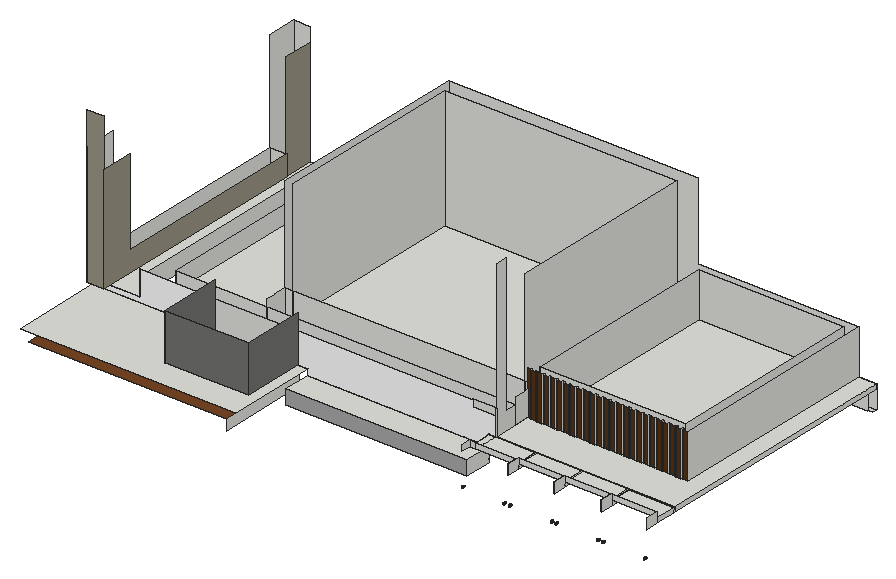
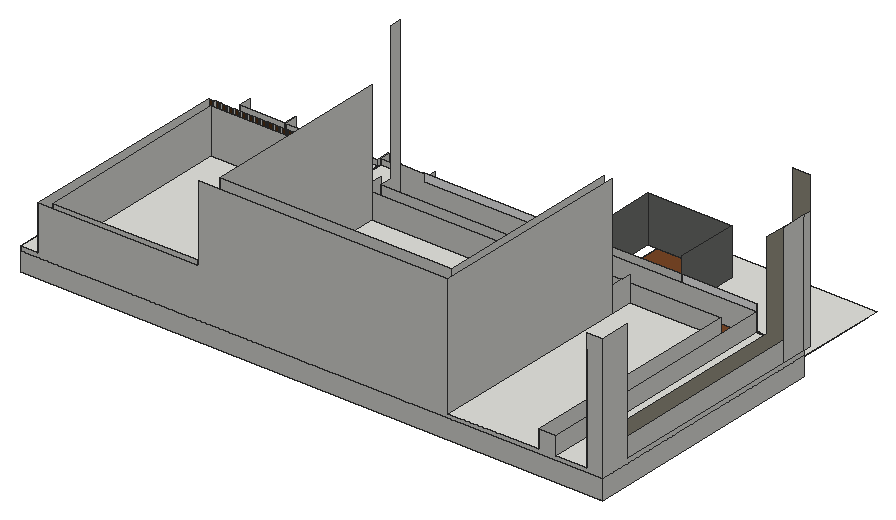
# SketchUp Ruby script. Lengths in inches.
U = 1.inch
M = Sketchup.active_model
def pt(a) = Geom::Point3d.new(a.map { |v| v * U })
def face(e, loops, mat)
  f = e.add_face(loops[0].map { |a| pt(a) })
  loops[1..].each { |l| e.add_face(l.map { |a| pt(a) }).erase! }
  f.material = f.back_material = mat if mat
  f
end
# faces: each face lists its corners as indices into pts; further lists are holes
def faces(e, pts, list, mat = nil) = list.each { |f| face(e, (f[0].is_a?(Array) ? f : [f]).map { |l| l.map { |i| pts[i] } }, mat) }
# xy, xz, yz: faces in a plane at the given z, y or x. An outline is a flat list of corners, or four numbers for a rectangle; further outlines are holes
def ring(l) = l.size == 4 ? [[l[0], l[1]], [l[2], l[1]], [l[2], l[3]], [l[0], l[3]]] : l.each_slice(2).to_a
def flat(e, list, mat, &to3) = list.each { |f| face(e, (f[0].is_a?(Array) ? f : [f]).map { |l| ring(l).map { |u, v| to3.(u, v) } }, mat) }
def xy(e, z, list, mat = nil) = flat(e, list, mat) { |x, y| [x, y, z] }
def xz(e, y, list, mat = nil) = flat(e, list, mat) { |x, z| [x, y, z] }
def yz(e, x, list, mat = nil) = flat(e, list, mat) { |y, z| [x, y, z] }
def lines(e, pts, list) = list.each { |a, b| e.add_line(pt(pts[a]), pt(pts[b])) }
# prism: a flat outline (further loops are holes) pulled along v
def prism(e, loops, v, mat = nil)
  f = face(e, loops, mat); d = Geom::Vector3d.new(v.map { |x| x * U })
  f.pushpull(f.normal.samedirection?(d) ? d.length : -d.length)
end
def box(e, o, s, mat = nil) = prism(e, [[o, [o[0] + s[0], o[1], o[2]], [o[0] + s[0], o[1] + s[1], o[2]], [o[0], o[1] + s[1], o[2]]]], [0, 0, s[2]], mat)
def at(x, y, z, deg = 0) = Geom::Transformation.translation(pt([x, y, z])) * Geom::Transformation.rotation(ORIGIN, Z_AXIS, deg.degrees)
def axes(o, x, y, z) = Geom::Transformation.new([*x, 0, *y, 0, *z, 0, *pt(o).to_a, 1])
def part(name) = M.definitions.add(name)
# library, detail: a bought-in or finely detailed component or shape, given as its bounding box
def library(name, o, s) = part(name).tap { |d| box(d.entities, o, s) }
def detail(e, o, s) = box(e.add_group.entities, o, s)
def put(e, d, t, mat = nil) = e.add_instance(d, t).tap { |i| i.material = mat if mat }
def group(e, t, mat = nil) = e.add_group.tap { |g| g.transformation = t; g.material = mat if mat }.entities
root = M.entities
M.materials.add("[0030_OldLace]").color = [86, 53, 24]
M.materials.add("[0128_White]").color = [255, 255, 255]
M.materials.add("[Color M03]").color = [170, 170, 170]
M.materials.add("[Concrete Tile]").color = [155, 150, 134]
M.materials.add("[Metal Seamed]").color = [116, 117, 113]
M.materials.add("[Wood Veneer 01]").color = [120, 70, 37]
xy(root,95.79,[[1564.1,846.1,1664.38,851.0625]])
xy(root,99.26,[[1501.42,810.97,1728.67,845.35]],"[Wood Veneer 01]")
xy(root,101.375,[[1425.1,845.35,1490.48,846.1],[1232.12,846.1,1232.12,1160.85,1960.87,1160.85,1960.87,1155.13,1237.84,1155.13,1237.84,851.0625,1425.1,851.0625,1425.1,846.1],[1425.1,846.1,1490.48,851.0625]])
xy(root,101.78,[[1254.78,845.35,1379.65,851.0625]])
xy(root,114.25,[[1243.06,732.28,1490.48,845.35]],"[Wood Veneer 01]")
xy(root,117.26,[[1501.42,810.97,1728.67,845.35]])
xy(root,125.1875,[[1232.12,732.28,1501.42,732.28,1501.42,845.35,1489.48,845.35,1489.48,767.72,1385.29,767.72,1385.29,845.35,1232.12,845.35],[1232.12,845.35,1501.42,846.1]])
xy(root,131.1875,[[1728.67,814.22,1729.13,844.47],[1729.13,814.22,1737.07,844.47],[1737.07,814.22,1786.72,844.47],[1787.65,817.6,1844.77,844.47],[1845.83,817.6,1902.82,844.47],
  [1904.13,817.6,1960.87,844.47],[1232.12,837.03,1252.87,845.35],[1728.67,844.47,1729.13,845.35],[1729.13,844.47,1737.07,845.35],[1737.07,844.47,1960.87,846.1],
  [1232.12,845.35,1252.87,846.1],[1252.87,845.35,1291.04,846.1],[1728.67,845.35,1729.13,846.1],[1729.13,845.35,1737.07,846.1],[1232.12,846.1,1252.87,877.14],
  [1252.87,846.1,1291.04,846.1,1291.04,1160.85,1252.24,1160.85,1252.24,1122.97,1252.87,1122.97],[1737.07,846.1,1960.87,846.1,1960.87,1160.85,1938.44,1160.85,1938.44,893.65,1932.29,893.65,1932.29,895.71,1930.13,895.71,1930.13,893.65,1923.98,893.65,1923.98,895.71,1921.82,895.71,1921.82,894.34,1915.67,894.34,1915.67,895.71,1913.51,895.71,1913.51,894.34,1907.36,894.34,1907.36,895.71,1905.19,895.71,1905.19,894.34,1899.04,894.34,1899.04,895.71,1896.88,895.71,1896.88,894.34,1890.73,894.34,1890.73,895.71,1888.57,895.71,1888.57,894.34,1882.42,894.34,1882.42,895.71,1880.26,895.71,1880.26,894.34,1874.11,894.34,1874.11,895.71,1871.94,895.71,1871.94,894.34,1865.79,894.34,1865.79,895.71,1863.63,895.71,1863.63,894.34,1857.48,894.34,1857.48,895.71,1855.32,895.71,1855.32,894.34,1849.17,894.34,1849.17,895.71,1847.01,895.71,1847.01,894.34,1840.86,894.34,1840.86,895.71,1838.69,895.71,1838.69,894.34,1832.54,894.34,1832.54,895.71,1830.38,895.71,1830.38,894.34,1824.23,894.34,1824.23,895.71,1822.07,895.71,1822.07,894.34,1815.92,894.34,1815.92,895.71,1813.76,895.71,1813.76,894.34,1807.61,894.34,1807.61,895.71,1805.44,895.71,1805.44,894.34,1799.29,894.34,1799.29,895.71,1797.13,895.71,1797.13,894.34,1790.98,894.34,1790.98,895.71,1788.82,895.71,1788.82,894.34,1782.67,894.34,1782.67,895.71,1780.51,895.71,1780.51,894.34,1774.36,894.34,1774.36,895.71,1772.19,895.71,1772.19,894.34,1766.04,894.34,1766.04,895.71,1763.88,895.71,1763.88,894.34,1757.73,894.34,1757.73,895.71,1755.57,895.71,1755.57,894.34,1749.42,894.34,1749.42,895.71,1747.26,895.71,1747.26,894.34,1741.11,894.34,1741.11,895.71,1737.07,895.71],[1232.12,877.14,1252.87,1122.97],[1311.45,877.14,1425.1,1160.85],[1425.1,877.14,1737.07,905.7],
  [1745.54,904.18,1927.22,1152.375],[1434.48,905.7,1724.81,1143.26]])
xz(root,767.72,[[1385.29,125.1875,1489.48,183.3125]],"[Metal Seamed]")
xz(root,799.91,[[1731.49,91.63,1731.78,91.67,1732.05,91.78,1732.29,91.96,1732.46,92.19,1732.58,92.46,1732.61,92.75,1732.58,93.04,1732.46,93.32,1732.29,93.55,1732.05,93.73,1731.78,93.84,1731.49,93.88,1731.2,93.84,1730.93,93.73,1730.69,93.55,1730.52,93.32,1730.4,93.04,1730.36,92.75,1730.4,92.46,1730.52,92.19,1730.69,91.96,1730.93,91.78,1731.2,91.67],[1783.68,91.63,1783.97,91.67,1784.24,91.78,1784.47,91.96,1784.65,92.19,1784.76,92.46,1784.8,92.75,1784.76,93.04,1784.65,93.32,1784.47,93.55,1784.24,93.73,1783.97,93.84,1783.68,93.88,1783.39,93.84,1783.11,93.73,1782.88,93.55,1782.7,93.32,1782.59,93.04,1782.55,92.75,1782.59,92.46,1782.7,92.19,1782.88,91.96,1783.11,91.78,1783.39,91.67],[1790.48,91.63,1790.77,91.67,1791.04,91.78,1791.27,91.96,1791.45,92.19,1791.56,92.46,1791.6,92.75,1791.56,93.04,1791.45,93.32,1791.27,93.55,1791.04,93.73,1790.77,93.84,1790.48,93.88,1790.1875,93.84,1789.92,93.73,1789.68,93.55,1789.5,93.32,1789.39,93.04,1789.35,92.75,1789.39,92.46,1789.5,92.19,1789.68,91.96,1789.92,91.78,1790.1875,91.67],[1842.67,91.63,1842.96,91.67,1843.23,91.78,1843.46,91.96,1843.64,92.19,1843.75,92.46,1843.79,92.75,1843.75,93.04,1843.64,93.32,1843.46,93.55,1843.23,93.73,1842.96,93.84,1842.67,93.88,1842.375,93.84,1842.1,93.73,1841.87,93.55,1841.69,93.32,1841.58,93.04,1841.54,92.75,1841.58,92.46,1841.69,92.19,1841.87,91.96,1842.1,91.78,1842.375,91.67],[1848.65,91.63,1848.94,91.67,1849.22,91.78,1849.45,91.96,1849.63,92.19,1849.74,92.46,1849.78,92.75,1849.74,93.04,1849.63,93.32,1849.45,93.55,1849.22,93.73,1848.94,93.84,1848.65,93.88,1848.36,93.84,1848.09,93.73,1847.86,93.55,1847.68,93.32,1847.57,93.04,1847.53,92.75,1847.57,92.46,1847.68,92.19,1847.86,91.96,1848.09,91.78,1848.36,91.67],
  [1900.84,91.63,1901.13,91.67,1901.4,91.78,1901.64,91.96,1901.82,92.19,1901.93,92.46,1901.97,92.75,1901.93,93.04,1901.82,93.32,1901.64,93.55,1901.4,93.73,1901.13,93.84,1900.84,93.88,1900.55,93.84,1900.28,93.73,1900.05,93.55,1899.87,93.32,1899.75,93.04,1899.72,92.75,1899.75,92.46,1899.87,92.19,1900.05,91.96,1900.28,91.78,1900.55,91.67],[1906.95,91.63,1907.25,91.67,1907.52,91.78,1907.75,91.96,1907.93,92.19,1908.04,92.46,1908.08,92.75,1908.04,93.04,1907.93,93.32,1907.75,93.55,1907.52,93.73,1907.25,93.84,1906.95,93.88,1906.66,93.84,1906.39,93.73,1906.16,93.55,1905.98,93.32,1905.87,93.04,1905.83,92.75,1905.87,92.46,1905.98,92.19,1906.16,91.96,1906.39,91.78,1906.66,91.67],[1959.14,91.63,1959.43,91.67,1959.7,91.78,1959.9375,91.96,1960.12,92.19,1960.23,92.46,1960.27,92.75,1960.23,93.04,1960.12,93.32,1959.9375,93.55,1959.7,93.73,1959.43,93.84,1959.14,93.88,1958.85,93.84,1958.58,93.73,1958.35,93.55,1958.17,93.32,1958.06,93.04,1958.02,92.75,1958.06,92.46,1958.17,92.19,1958.35,91.96,1958.58,91.78,1958.85,91.67]])
xz(root,810.97,[[1501.42,99.26,1728.67,117.26]],"[Color M03]")
xz(root,814.22,[[1728.67,131.1875,1737.07,138.0625],[1737.07,131.1875,1786.72,138.0625]])
xz(root,817.6,[[1787.65,131.1875,1844.77,138.0625],[1845.83,131.1875,1902.82,138.0625],[1904.13,131.1875,1960.87,138.0625]])
xz(root,837.03,[[1232.12,131.1875,1252.87,324.5625]],"[Concrete Tile]")
xz(root,845.35,[[1501.42,99.26,1728.67,117.26],[1385.29,125.1875,1489.48,162.75]])
xz(root,845.35,[[1501.42,117.26,1728.67,117.26,1728.67,131.1875,1737.07,131.1875,1737.07,154.75,1707.86,154.75,1707.86,162.75,1489.48,162.75,1489.48,125.1875,1501.42,125.1875],[1232.12,125.1875,1385.29,125.1875,1385.29,162.75,1291.04,162.75,1291.04,131.1875,1232.12,131.1875]],"[0128_White]")
xz(root,846.1,[[1232.12,125.1875,1232.12,131.1875,1291.04,131.1875,1291.04,153.5625,1707.86,153.5625,1707.86,163,1737.07,163,1737.07,131.1875,1728.67,131.1875,1728.67,125.1875]])
xz(root,851.0625,[[1254.78,101.375,1379.65,101.78]])
xz(root,877.14,[[1311.45,131.1875,1425.1,153.5625],[1425.1,131.1875,1737.07,153.5625]])
xz(root,893.65,[[1923.98,131.1875,1930.13,186.75],[1932.29,131.1875,1938.44,186.75]],"[0030_OldLace]")
xz(root,894.34,[[1741.11,131.1875,1747.26,186.75],[1749.42,131.1875,1755.57,186.75],[1757.73,131.1875,1763.88,186.75],[1766.04,131.1875,1772.19,186.75],[1774.36,131.1875,1780.51,186.75],
  [1782.67,131.1875,1788.82,186.75],[1790.98,131.1875,1797.13,186.75],[1799.29,131.1875,1805.44,186.75],[1807.61,131.1875,1813.76,186.75],[1815.92,131.1875,1822.07,186.75],
  [1824.23,131.1875,1830.38,186.75],[1832.54,131.1875,1838.69,186.75],[1840.86,131.1875,1847.01,186.75],[1849.17,131.1875,1855.32,186.75],[1857.48,131.1875,1863.63,186.75],
  [1865.79,131.1875,1871.94,186.75],[1874.11,131.1875,1880.26,186.75],[1882.42,131.1875,1888.57,186.75],[1890.73,131.1875,1896.88,186.75],[1899.04,131.1875,1905.19,186.75],
  [1907.36,131.1875,1913.51,186.75],[1915.67,131.1875,1921.82,186.75]],"[0030_OldLace]")
xz(root,895.71,[[1737.07,131.1875,1741.11,186.75],[1747.26,131.1875,1749.42,186.75],[1755.57,131.1875,1757.73,186.75],[1763.88,131.1875,1766.04,186.75],[1772.19,131.1875,1774.36,186.75],
  [1780.51,131.1875,1782.67,186.75],[1788.82,131.1875,1790.98,186.75],[1797.13,131.1875,1799.29,186.75],[1805.44,131.1875,1807.61,186.75],[1813.76,131.1875,1815.92,186.75],
  [1822.07,131.1875,1824.23,186.75],[1830.38,131.1875,1832.54,186.75],[1838.69,131.1875,1840.86,186.75],[1847.01,131.1875,1849.17,186.75],[1855.32,131.1875,1857.48,186.75],
  [1863.63,131.1875,1865.79,186.75],[1871.94,131.1875,1874.11,186.75],[1880.26,131.1875,1882.42,186.75],[1888.57,131.1875,1890.73,186.75],[1896.88,131.1875,1899.04,186.75],
  [1905.19,131.1875,1907.36,186.75],[1913.51,131.1875,1915.67,186.75],[1921.82,131.1875,1923.98,186.75],[1930.13,131.1875,1932.29,186.75]],"[0030_OldLace]")
xz(root,904.18,[[1745.54,131.1875,1927.22,186.75]])
xz(root,905.7,[[1425.1,131.1875,1434.48,162.75],[1434.48,131.1875,1724.81,162.75],[1724.81,131.1875,1737.07,162.75]])
xz(root,1122.97,[[1232.12,131.1875,1252.24,156.5],[1252.24,131.1875,1252.87,156.5]])
xz(root,1143.26,[[1434.48,131.1875,1724.81,282.75]])
xz(root,1152.375,[[1745.54,131.1875,1927.22,186.75]])
xz(root,1155.13,[[1237.84,101.375,1955.15,125.1875]])
xz(root,1160.85,[[1232.12,101.375,1960.87,125.1875],[1232.12,125.1875,1232.12,282.75,1252.24,282.75,1252.24,131.1875,1291.04,131.1875,1291.04,153.5625,1311.45,153.5625,1311.45,131.1875,1425.1,131.1875,1425.1,282.75,1737.07,282.75,1737.07,186.75,1938.44,186.75,1938.44,131.1875,1960.87,131.1875,1960.87,125.1875]])
yz(root,1232.12,[[846.1,101.375,1160.85,125.1875],[845.35,125.1875,846.1,131.1875],[846.1,125.1875,846.1,131.1875,1122.97,131.1875,1122.97,282.75,1160.85,282.75,1160.85,125.1875],[837.03,131.1875,845.35,282.75],[845.35,131.1875,877.14,282.75],
  [877.14,131.1875,1122.97,156.5]])
yz(root,1237.84,[[851.0625,101.375,1155.13,125.1875]])
yz(root,1252.24,[[1122.97,131.1875,1160.85,264.75]],"[Concrete Tile]")
yz(root,1252.87,[[837.03,131.1875,1122.97,131.1875,1122.97,156.5,877.14,156.5,877.14,264.75,837.03,264.75]],"[Concrete Tile]")
yz(root,1291.04,[[845.35,131.1875,846.1,162.75],[846.1,131.1875,1160.85,153.5625]])
yz(root,1311.45,[[877.14,131.1875,1160.85,153.5625]])
yz(root,1385.29,[[767.72,125.1875,845.35,183.3125]],"[Metal Seamed]")
yz(root,1425.1,[[877.14,131.1875,877.14,162.125,888.95,162.125,888.95,162.75,905.7,162.75,905.7,131.1875],[905.7,131.1875,1160.85,282.75]])
yz(root,1434.48,[[905.7,131.1875,1143.26,282.75]])
yz(root,1489.48,[[767.72,125.1875,845.35,183.3125]],"[Metal Seamed]")
yz(root,1490.48,[[732.28,101.375,845.35,114.25]])
yz(root,1724.81,[[905.7,131.1875,1143.26,282.75]])
yz(root,1728.67,[[810.97,99.26,844.47,117.26],[844.47,99.26,845.35,117.26],[844.47,117.26,845.35,125.1875],[844.47,125.1875,845.35,131.1875],[845.35,125.1875,846.1,131.1875],
  [801.78,131.1875,814.22,138.0625]])
yz(root,1737.07,[[845.35,131.1875,846.1,163],[846.1,131.1875,877.14,131.1875,877.14,153.5625,861.24,153.5625,861.24,324.5625,846.1,324.5625],[877.14,131.1875,895.71,131.1875,895.71,162.75,890.39,162.75,890.39,162.125,877.14,162.125],[895.71,131.1875,905.7,162.75]])
yz(root,1741.11,[[894.34,131.1875,895.71,186.75]])
yz(root,1745.54,[[904.18,131.1875,905.7,186.75],[905.7,131.1875,1152.375,186.75]])
yz(root,1747.26,[[894.34,131.1875,895.71,186.75]])
yz(root,1749.42,[[894.34,131.1875,895.71,186.75]])
yz(root,1755.57,[[894.34,131.1875,895.71,186.75]])
yz(root,1757.73,[[894.34,131.1875,895.71,186.75]])
yz(root,1763.88,[[894.34,131.1875,895.71,186.75]])
yz(root,1766.04,[[894.34,131.1875,895.71,186.75]])
yz(root,1772.19,[[894.34,131.1875,895.71,186.75]])
yz(root,1774.36,[[894.34,131.1875,895.71,186.75]])
yz(root,1780.51,[[894.34,131.1875,895.71,186.75]])
yz(root,1782.67,[[894.34,131.1875,895.71,186.75]])
yz(root,1786.72,[[801.78,125.1875,814.22,138.0625],[814.22,125.1875,844.47,131.1875]])
yz(root,1787.65,[[801.78,125.1875,817.6,138.0625],[817.6,125.1875,844.47,131.1875]])
yz(root,1788.82,[[894.34,131.1875,895.71,186.75]])
yz(root,1790.98,[[894.34,131.1875,895.71,186.75]])
yz(root,1797.13,[[894.34,131.1875,895.71,186.75]])
yz(root,1799.29,[[894.34,131.1875,895.71,186.75]])
yz(root,1805.44,[[894.34,131.1875,895.71,186.75]])
yz(root,1807.61,[[894.34,131.1875,895.71,186.75]])
yz(root,1813.76,[[894.34,131.1875,895.71,186.75]])
yz(root,1815.92,[[894.34,131.1875,895.71,186.75]])
yz(root,1822.07,[[894.34,131.1875,895.71,186.75]])
yz(root,1824.23,[[894.34,131.1875,895.71,186.75]])
yz(root,1830.38,[[894.34,131.1875,895.71,186.75]])
yz(root,1832.54,[[894.34,131.1875,895.71,186.75]])
yz(root,1838.69,[[894.34,131.1875,895.71,186.75]])
yz(root,1840.86,[[894.34,131.1875,895.71,186.75]])
yz(root,1844.77,[[801.78,125.1875,817.6,138.0625],[817.6,125.1875,844.47,131.1875]])
yz(root,1845.83,[[801.78,125.1875,817.6,138.0625],[817.6,125.1875,844.47,131.1875]])
yz(root,1847.01,[[894.34,131.1875,895.71,186.75]])
yz(root,1849.17,[[894.34,131.1875,895.71,186.75]])
yz(root,1855.32,[[894.34,131.1875,895.71,186.75]])
yz(root,1857.48,[[894.34,131.1875,895.71,186.75]])
yz(root,1863.63,[[894.34,131.1875,895.71,186.75]])
yz(root,1865.79,[[894.34,131.1875,895.71,186.75]])
yz(root,1871.94,[[894.34,131.1875,895.71,186.75]])
yz(root,1874.11,[[894.34,131.1875,895.71,186.75]])
yz(root,1880.26,[[894.34,131.1875,895.71,186.75]])
yz(root,1882.42,[[894.34,131.1875,895.71,186.75]])
yz(root,1888.57,[[894.34,131.1875,895.71,186.75]])
yz(root,1890.73,[[894.34,131.1875,895.71,186.75]])
yz(root,1896.88,[[894.34,131.1875,895.71,186.75]])
yz(root,1899.04,[[894.34,131.1875,895.71,186.75]])
yz(root,1902.82,[[801.78,125.1875,817.6,138.0625],[817.6,125.1875,844.47,131.1875]])
yz(root,1904.13,[[801.78,125.1875,817.6,138.0625],[817.6,125.1875,844.47,131.1875]])
yz(root,1905.19,[[894.34,131.1875,895.71,186.75]])
yz(root,1907.36,[[894.34,131.1875,895.71,186.75]])
yz(root,1913.51,[[894.34,131.1875,895.71,186.75]])
yz(root,1915.67,[[894.34,131.1875,895.71,186.75]],"[0030_OldLace]")
yz(root,1921.82,[[894.34,131.1875,895.71,186.75]])
yz(root,1923.98,[[893.65,131.1875,895.71,186.75]],"[0030_OldLace]")
yz(root,1927.22,[[904.18,131.1875,1152.375,186.75]])
yz(root,1930.13,[[893.65,131.1875,895.71,186.75]])
yz(root,1932.29,[[893.65,131.1875,895.71,186.75]],"[0030_OldLace]")
yz(root,1938.44,[[893.65,131.1875,1160.85,186.75]])
yz(root,1960.87,[[801.78,125.1875,817.6,138.0625],[817.6,125.1875,844.47,131.1875],[844.47,125.1875,846.1,131.1875],[846.1,125.1875,1160.85,131.1875]])
p = [[1731.2,801.78,91.67],[1731.49,801.78,91.63],[1731.49,799.91,91.63],[1731.2,799.91,91.67],[1731.78,801.78,91.67],[1731.78,799.91,91.67],
  [1783.39,801.78,91.67],[1783.68,801.78,91.63],[1783.68,799.91,91.63],[1783.39,799.91,91.67],[1783.97,801.78,91.67],[1783.97,799.91,91.67],
  [1790.1875,801.78,91.67],[1790.48,801.78,91.63],[1790.48,799.91,91.63],[1790.1875,799.91,91.67],[1790.77,801.78,91.67],[1790.77,799.91,91.67],
  [1842.375,801.78,91.67],[1842.67,801.78,91.63],[1842.67,799.91,91.63],[1842.375,799.91,91.67],[1842.96,801.78,91.67],[1842.96,799.91,91.67],
  [1848.36,801.78,91.67],[1848.65,801.78,91.63],[1848.65,799.91,91.63],[1848.36,799.91,91.67],[1848.94,801.78,91.67],[1848.94,799.91,91.67],
  [1900.55,801.78,91.67],[1900.84,801.78,91.63],[1900.84,799.91,91.63],[1900.55,799.91,91.67],[1901.13,801.78,91.67],[1901.13,799.91,91.67],
  [1906.66,801.78,91.67],[1906.95,801.78,91.63],[1906.95,799.91,91.63],[1906.66,799.91,91.67],[1907.25,801.78,91.67],[1907.25,799.91,91.67],
  [1958.85,801.78,91.67],[1959.14,801.78,91.63],[1959.14,799.91,91.63],[1958.85,799.91,91.67],[1959.43,801.78,91.67],[1959.43,799.91,91.67],
  [1730.93,801.78,91.78],[1730.93,799.91,91.78],[1732.05,801.78,91.78],[1732.05,799.91,91.78],[1783.11,801.78,91.78],[1783.11,799.91,91.78],
  [1784.24,801.78,91.78],[1784.24,799.91,91.78],[1789.92,801.78,91.78],[1789.92,799.91,91.78],[1791.04,801.78,91.78],[1791.04,799.91,91.78],
  [1842.1,801.78,91.78],[1842.1,799.91,91.78],[1843.23,801.78,91.78],[1843.23,799.91,91.78],[1848.09,801.78,91.78],[1848.09,799.91,91.78],
  [1849.22,801.78,91.78],[1849.22,799.91,91.78],[1900.28,801.78,91.78],[1900.28,799.91,91.78],[1901.4,801.78,91.78],[1901.4,799.91,91.78],
  [1906.39,801.78,91.78],[1906.39,799.91,91.78],[1907.52,801.78,91.78],[1907.52,799.91,91.78],[1958.58,801.78,91.78],[1958.58,799.91,91.78],
  [1959.7,801.78,91.78],[1959.7,799.91,91.78],[1730.69,801.78,91.96],[1730.69,799.91,91.96],[1732.29,801.78,91.96],[1732.29,799.91,91.96],
  [1782.88,801.78,91.96],[1782.88,799.91,91.96],[1784.47,801.78,91.96],[1784.47,799.91,91.96],[1789.68,801.78,91.96],[1789.68,799.91,91.96],
  [1791.27,801.78,91.96],[1791.27,799.91,91.96],[1841.87,801.78,91.96],[1841.87,799.91,91.96],[1843.46,801.78,91.96],[1843.46,799.91,91.96],
  [1847.86,801.78,91.96],[1847.86,799.91,91.96],[1849.45,801.78,91.96],[1849.45,799.91,91.96],[1900.05,801.78,91.96],[1900.05,799.91,91.96],
  [1901.64,801.78,91.96],[1901.64,799.91,91.96],[1906.16,801.78,91.96],[1906.16,799.91,91.96],[1907.75,801.78,91.96],[1907.75,799.91,91.96],
  [1958.35,801.78,91.96],[1958.35,799.91,91.96],[1959.9375,801.78,91.96],[1959.9375,799.91,91.96],[1730.52,801.78,92.19],[1730.52,799.91,92.19],
  [1732.46,801.78,92.19],[1732.46,799.91,92.19],[1782.7,801.78,92.19],[1782.7,799.91,92.19],[1784.65,801.78,92.19],[1784.65,799.91,92.19],
  [1789.5,801.78,92.19],[1789.5,799.91,92.19],[1791.45,801.78,92.19],[1791.45,799.91,92.19],[1841.69,801.78,92.19],[1841.69,799.91,92.19],
  [1843.64,801.78,92.19],[1843.64,799.91,92.19],[1847.68,801.78,92.19],[1847.68,799.91,92.19],[1849.63,801.78,92.19],[1849.63,799.91,92.19],
  [1899.87,801.78,92.19],[1899.87,799.91,92.19],[1901.82,801.78,92.19],[1901.82,799.91,92.19],[1905.98,801.78,92.19],[1905.98,799.91,92.19],
  [1907.93,801.78,92.19],[1907.93,799.91,92.19],[1958.17,801.78,92.19],[1958.17,799.91,92.19],[1960.12,801.78,92.19],[1960.12,799.91,92.19],
  [1730.4,801.78,92.46],[1730.4,799.91,92.46],[1732.58,801.78,92.46],[1732.58,799.91,92.46],[1782.59,801.78,92.46],[1782.59,799.91,92.46],
  [1784.76,801.78,92.46],[1784.76,799.91,92.46],[1789.39,801.78,92.46],[1789.39,799.91,92.46],[1791.56,801.78,92.46],[1791.56,799.91,92.46],
  [1841.58,801.78,92.46],[1841.58,799.91,92.46],[1843.75,801.78,92.46],[1843.75,799.91,92.46],[1847.57,801.78,92.46],[1847.57,799.91,92.46],
  [1849.74,801.78,92.46],[1849.74,799.91,92.46],[1899.75,801.78,92.46],[1899.75,799.91,92.46],[1901.93,801.78,92.46],[1901.93,799.91,92.46],
  [1905.87,801.78,92.46],[1905.87,799.91,92.46],[1908.04,801.78,92.46],[1908.04,799.91,92.46],[1958.06,801.78,92.46],[1958.06,799.91,92.46],
  [1960.23,801.78,92.46],[1960.23,799.91,92.46],[1730.36,801.78,92.75],[1730.36,799.91,92.75],[1732.61,801.78,92.75],[1732.61,799.91,92.75],
  [1782.55,801.78,92.75],[1782.55,799.91,92.75],[1784.8,801.78,92.75],[1784.8,799.91,92.75],[1789.35,801.78,92.75],[1789.35,799.91,92.75],
  [1791.6,801.78,92.75],[1791.6,799.91,92.75],[1841.54,801.78,92.75],[1841.54,799.91,92.75],[1843.79,801.78,92.75],[1843.79,799.91,92.75],
  [1847.53,801.78,92.75],[1847.53,799.91,92.75],[1849.78,801.78,92.75],[1849.78,799.91,92.75],[1899.72,801.78,92.75],[1899.72,799.91,92.75],
  [1901.97,801.78,92.75],[1901.97,799.91,92.75],[1905.83,801.78,92.75],[1905.83,799.91,92.75],[1908.08,801.78,92.75],[1908.08,799.91,92.75],
  [1958.02,801.78,92.75],[1958.02,799.91,92.75],[1960.27,801.78,92.75],[1960.27,799.91,92.75],[1730.4,801.78,93.04],[1730.4,799.91,93.04],
  [1732.58,801.78,93.04],[1732.58,799.91,93.04],[1782.59,801.78,93.04],[1782.59,799.91,93.04],[1784.76,801.78,93.04],[1784.76,799.91,93.04],
  [1789.39,801.78,93.04],[1789.39,799.91,93.04],[1791.56,801.78,93.04],[1791.56,799.91,93.04],[1841.58,801.78,93.04],[1841.58,799.91,93.04],
  [1843.75,801.78,93.04],[1843.75,799.91,93.04],[1847.57,801.78,93.04],[1847.57,799.91,93.04],[1849.74,801.78,93.04],[1849.74,799.91,93.04],
  [1899.75,801.78,93.04],[1899.75,799.91,93.04],[1901.93,801.78,93.04],[1901.93,799.91,93.04],[1905.87,801.78,93.04],[1905.87,799.91,93.04],
  [1908.04,801.78,93.04],[1908.04,799.91,93.04],[1958.06,801.78,93.04],[1958.06,799.91,93.04],[1960.23,801.78,93.04],[1960.23,799.91,93.04],
  [1730.52,801.78,93.32],[1730.52,799.91,93.32],[1732.46,801.78,93.32],[1732.46,799.91,93.32],[1782.7,801.78,93.32],[1782.7,799.91,93.32],
  [1784.65,801.78,93.32],[1784.65,799.91,93.32],[1789.5,801.78,93.32],[1789.5,799.91,93.32],[1791.45,801.78,93.32],[1791.45,799.91,93.32],
  [1841.69,801.78,93.32],[1841.69,799.91,93.32],[1843.64,801.78,93.32],[1843.64,799.91,93.32],[1847.68,801.78,93.32],[1847.68,799.91,93.32],
  [1849.63,801.78,93.32],[1849.63,799.91,93.32],[1899.87,801.78,93.32],[1899.87,799.91,93.32],[1901.82,801.78,93.32],[1901.82,799.91,93.32],
  [1905.98,801.78,93.32],[1905.98,799.91,93.32],[1907.93,801.78,93.32],[1907.93,799.91,93.32],[1958.17,801.78,93.32],[1958.17,799.91,93.32],
  [1960.12,801.78,93.32],[1960.12,799.91,93.32],[1730.69,801.78,93.55],[1730.69,799.91,93.55],[1732.29,801.78,93.55],[1732.29,799.91,93.55],
  [1782.88,801.78,93.55],[1782.88,799.91,93.55],[1784.47,801.78,93.55],[1784.47,799.91,93.55],[1789.68,801.78,93.55],[1789.68,799.91,93.55],
  [1791.27,801.78,93.55],[1791.27,799.91,93.55],[1841.87,801.78,93.55],[1841.87,799.91,93.55],[1843.46,801.78,93.55],[1843.46,799.91,93.55],
  [1847.86,801.78,93.55],[1847.86,799.91,93.55],[1849.45,801.78,93.55],[1849.45,799.91,93.55],[1900.05,801.78,93.55],[1900.05,799.91,93.55],
  [1901.64,801.78,93.55],[1901.64,799.91,93.55],[1906.16,801.78,93.55],[1906.16,799.91,93.55],[1907.75,801.78,93.55],[1907.75,799.91,93.55],
  [1958.35,801.78,93.55],[1958.35,799.91,93.55],[1959.9375,801.78,93.55],[1959.9375,799.91,93.55],[1730.93,801.78,93.73],[1730.93,799.91,93.73],
  [1732.05,801.78,93.73],[1732.05,799.91,93.73],[1783.11,801.78,93.73],[1783.11,799.91,93.73],[1784.24,801.78,93.73],[1784.24,799.91,93.73],
  [1789.92,801.78,93.73],[1789.92,799.91,93.73],[1791.04,801.78,93.73],[1791.04,799.91,93.73],[1842.1,801.78,93.73],[1842.1,799.91,93.73],
  [1843.23,801.78,93.73],[1843.23,799.91,93.73],[1848.09,801.78,93.73],[1848.09,799.91,93.73],[1849.22,801.78,93.73],[1849.22,799.91,93.73],
  [1900.28,801.78,93.73],[1900.28,799.91,93.73],[1901.4,801.78,93.73],[1901.4,799.91,93.73],[1906.39,801.78,93.73],[1906.39,799.91,93.73],
  [1907.52,801.78,93.73],[1907.52,799.91,93.73],[1958.58,801.78,93.73],[1958.58,799.91,93.73],[1959.7,801.78,93.73],[1959.7,799.91,93.73],
  [1731.2,801.78,93.84],[1731.2,799.91,93.84],[1731.78,801.78,93.84],[1731.78,799.91,93.84],[1783.39,801.78,93.84],[1783.39,799.91,93.84],
  [1783.97,801.78,93.84],[1783.97,799.91,93.84],[1790.1875,801.78,93.84],[1790.1875,799.91,93.84],[1790.77,801.78,93.84],[1790.77,799.91,93.84],
  [1842.375,801.78,93.84],[1842.375,799.91,93.84],[1842.96,801.78,93.84],[1842.96,799.91,93.84],[1848.36,801.78,93.84],[1848.36,799.91,93.84],
  [1848.94,801.78,93.84],[1848.94,799.91,93.84],[1900.55,801.78,93.84],[1900.55,799.91,93.84],[1901.13,801.78,93.84],[1901.13,799.91,93.84],
  [1906.66,801.78,93.84],[1906.66,799.91,93.84],[1907.25,801.78,93.84],[1907.25,799.91,93.84],[1958.85,801.78,93.84],[1958.85,799.91,93.84],
  [1959.43,801.78,93.84],[1959.43,799.91,93.84],[1731.49,801.78,93.88],[1731.49,799.91,93.88],[1783.68,801.78,93.88],[1783.68,799.91,93.88],
  [1790.48,801.78,93.88],[1790.48,799.91,93.88],[1842.67,801.78,93.88],[1842.67,799.91,93.88],[1848.65,801.78,93.88],[1848.65,799.91,93.88],
  [1900.84,801.78,93.88],[1900.84,799.91,93.88],[1906.95,801.78,93.88],[1906.95,799.91,93.88],[1959.14,801.78,93.88],[1959.14,799.91,93.88]]
faces(root,p,[[0,1,2,3],[1,4,5,2],[6,7,8,9],[7,10,11,8],[12,13,14,15],[13,16,17,14],[18,19,20,21],[19,22,23,20],
  [24,25,26,27],[25,28,29,26],[30,31,32,33],[31,34,35,32],[36,37,38,39],[37,40,41,38],[42,43,44,45],[43,46,47,44],
  [48,0,3,49],[4,50,51,5],[52,6,9,53],[10,54,55,11],[56,12,15,57],[16,58,59,17],[60,18,21,61],[22,62,63,23],
  [64,24,27,65],[28,66,67,29],[68,30,33,69],[34,70,71,35],[72,36,39,73],[40,74,75,41],[76,42,45,77],[46,78,79,47],
  [80,48,49,81],[50,82,83,51],[84,52,53,85],[54,86,87,55],[88,56,57,89],[58,90,91,59],[92,60,61,93],[62,94,95,63],
  [96,64,65,97],[66,98,99,67],[100,68,69,101],[70,102,103,71],[104,72,73,105],[74,106,107,75],[108,76,77,109],[78,110,111,79],
  [112,80,81,113],[82,114,115,83],[116,84,85,117],[86,118,119,87],[120,88,89,121],[90,122,123,91],[124,92,93,125],[94,126,127,95],
  [128,96,97,129],[98,130,131,99],[132,100,101,133],[102,134,135,103],[136,104,105,137],[106,138,139,107],[140,108,109,141],[110,142,143,111],
  [144,112,113,145],[114,146,147,115],[148,116,117,149],[118,150,151,119],[152,120,121,153],[122,154,155,123],[156,124,125,157],[126,158,159,127],
  [160,128,129,161],[130,162,163,131],[164,132,133,165],[134,166,167,135],[168,136,137,169],[138,170,171,139],[172,140,141,173],[142,174,175,143],
  [176,144,145,177],[146,178,179,147],[180,148,149,181],[150,182,183,151],[184,152,153,185],[154,186,187,155],[188,156,157,189],[158,190,191,159],
  [192,160,161,193],[162,194,195,163],[196,164,165,197],[166,198,199,167],[200,168,169,201],[170,202,203,171],[204,172,173,205],[174,206,207,175],
  [208,176,177,209],[178,210,211,179],[212,180,181,213],[182,214,215,183],[216,184,185,217],[186,218,219,187],[220,188,189,221],[190,222,223,191],
  [224,192,193,225],[194,226,227,195],[228,196,197,229],[198,230,231,199],[232,200,201,233],[202,234,235,203],[236,204,205,237],[206,238,239,207],
  [240,208,209,241],[210,242,243,211],[244,212,213,245],[214,246,247,215],[248,216,217,249],[218,250,251,219],[252,220,221,253],[222,254,255,223],
  [256,224,225,257],[226,258,259,227],[260,228,229,261],[230,262,263,231],[264,232,233,265],[234,266,267,235],[268,236,237,269],[238,270,271,239],
  [272,240,241,273],[242,274,275,243],[276,244,245,277],[246,278,279,247],[280,248,249,281],[250,282,283,251],[284,252,253,285],[254,286,287,255],
  [288,256,257,289],[258,290,291,259],[292,260,261,293],[262,294,295,263],[296,264,265,297],[266,298,299,267],[300,268,269,301],[270,302,303,271],
  [304,272,273,305],[274,306,307,275],[308,276,277,309],[278,310,311,279],[312,280,281,313],[282,314,315,283],[316,284,285,317],[286,318,319,287],
  [320,288,289,321],[290,322,323,291],[324,292,293,325],[294,326,327,295],[328,296,297,329],[298,330,331,299],[332,300,301,333],[302,334,335,303],
  [336,304,305,337],[306,338,339,307],[340,308,309,341],[310,342,343,311],[344,312,313,345],[314,346,347,315],[348,316,317,349],[318,350,351,319],
  [352,320,321,353],[322,354,355,323],[356,324,325,357],[326,358,359,327],[360,328,329,361],[330,362,363,331],[364,332,333,365],[334,366,367,335],
  [368,336,337,369],[338,368,369,339],[370,340,341,371],[342,370,371,343],[372,344,345,373],[346,372,373,347],[374,348,349,375],[350,374,375,351],
  [376,352,353,377],[354,376,377,355],[378,356,357,379],[358,378,379,359],[380,360,361,381],[362,380,381,363],[382,364,365,383],[366,382,383,367]])
